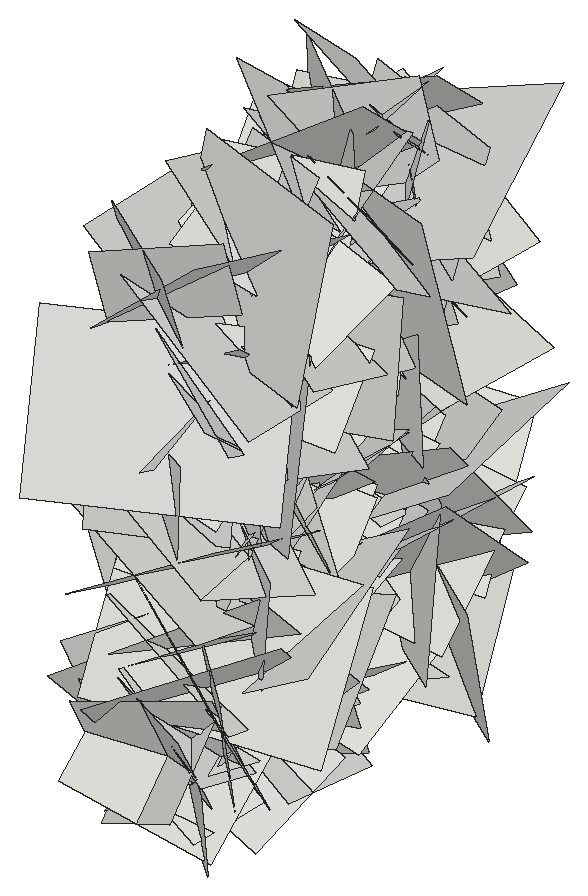
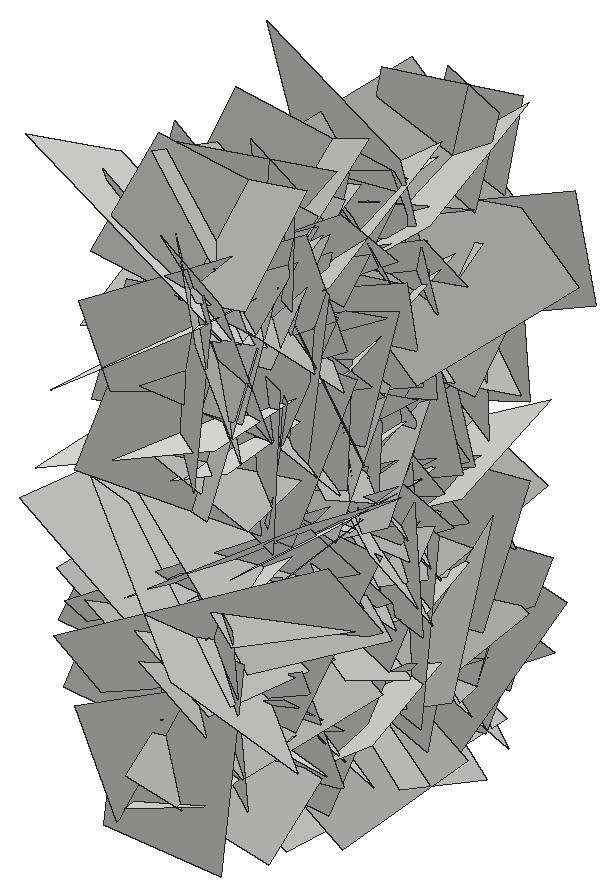
# SketchUp Ruby script. Lengths in inches.
U = 1.inch
M = Sketchup.active_model
def pt(a) = Geom::Point3d.new(a.map { |v| v * U })
def face(e, loops, mat)
  f = e.add_face(loops[0].map { |a| pt(a) })
  loops[1..].each { |l| e.add_face(l.map { |a| pt(a) }).erase! }
  f.material = f.back_material = mat if mat
  f
end
# faces: each face lists its corners as indices into pts; further lists are holes
def faces(e, pts, list, mat = nil) = list.each { |f| face(e, (f[0].is_a?(Array) ? f : [f]).map { |l| l.map { |i| pts[i] } }, mat) }
# xy, xz, yz: faces in a plane at the given z, y or x. An outline is a flat list of corners, or four numbers for a rectangle; further outlines are holes
def ring(l) = l.size == 4 ? [[l[0], l[1]], [l[2], l[1]], [l[2], l[3]], [l[0], l[3]]] : l.each_slice(2).to_a
def flat(e, list, mat, &to3) = list.each { |f| face(e, (f[0].is_a?(Array) ? f : [f]).map { |l| ring(l).map { |u, v| to3.(u, v) } }, mat) }
def xy(e, z, list, mat = nil) = flat(e, list, mat) { |x, y| [x, y, z] }
def xz(e, y, list, mat = nil) = flat(e, list, mat) { |x, z| [x, y, z] }
def yz(e, x, list, mat = nil) = flat(e, list, mat) { |y, z| [x, y, z] }
def lines(e, pts, list) = list.each { |a, b| e.add_line(pt(pts[a]), pt(pts[b])) }
# prism: a flat outline (further loops are holes) pulled along v
def prism(e, loops, v, mat = nil)
  f = face(e, loops, mat); d = Geom::Vector3d.new(v.map { |x| x * U })
  f.pushpull(f.normal.samedirection?(d) ? d.length : -d.length)
end
def box(e, o, s, mat = nil) = prism(e, [[o, [o[0] + s[0], o[1], o[2]], [o[0] + s[0], o[1] + s[1], o[2]], [o[0], o[1] + s[1], o[2]]]], [0, 0, s[2]], mat)
def at(x, y, z, deg = 0) = Geom::Transformation.translation(pt([x, y, z])) * Geom::Transformation.rotation(ORIGIN, Z_AXIS, deg.degrees)
def axes(o, x, y, z) = Geom::Transformation.new([*x, 0, *y, 0, *z, 0, *pt(o).to_a, 1])
def part(name) = M.definitions.add(name)
# library, detail: a bought-in or finely detailed component or shape, given as its bounding box
def library(name, o, s) = part(name).tap { |d| box(d.entities, o, s) }
def detail(e, o, s) = box(e.add_group.entities, o, s)
def put(e, d, t, mat = nil) = e.add_instance(d, t).tap { |i| i.material = mat if mat }
def group(e, t, mat = nil) = e.add_group.tap { |g| g.transformation = t; g.material = mat if mat }.entities
root = M.entities
c1 = part("Component\#6")
p = [[0.01,0,0],[0,3.24,4.54],[4.32,3.24,4.54],[4.33,0,0]]
faces(c1.entities,p,[[0,1,2,3]])
put(root,c1,axes([424.49,182.77,28.15],[0.11013,-1.0722,-0.31704],[0.03816,-0.31503,1.07721],[-1.18456,-0.10983,0.00522]))
put(root,c1,axes([424.49,185.38,28.27],[0.28552,-0.8956,-0.93898],[0.07116,-0.9481,0.92355],[-1.37362,-0.23528,-0.14733]))
put(root,c1,axes([420.52,175.43,34.87],[-0.0411,0.62613,0.35799],[-0.03637,0.3565,-0.62724],[0.76365,0.05068,-0.01061]))
put(root,c1,axes([420.52,173.67,32.24],[-0.05341,-0.65994,-0.37026],[-0.06447,-0.36634,0.66124],[0.79951,-0.07362,0.02859]))
put(root,c1,axes([424.49,174.01,26.46],[0.07872,-0.97306,0.24072],[-0.0738,0.23579,0.97461],[-1.05998,-0.08868,-0.04998]))
put(root,c1,axes([424.49,170.16,39.2],[0.24703,1.2789,-0.21613],[0.13589,-0.24123,-1.28918],[-1.36812,0.20696,-0.16707]))
put(root,c1,axes([420.52,173.15,22.23],[0.01199,-0.5915,0.12784],[0.10227,0.12799,0.58366],[0.63327,-0.00947,-0.09668]))
put(root,c1,axes([420.52,174.375,32.02],[-0.18574,0.64681,-0.5499],[-0.00393,-0.56207,-0.65994],[0.8999,0.13105,-0.11638]))
put(root,c1,axes([420.52,171.42,39.46],[0.01769,0.21401,-0.61924],[0.03571,-0.6189,-0.21298],[0.69357,0.02641,0.02676]))
put(root,c1,axes([420.52,180.11,41],[-0.0874,0.13713,-0.78202],[-0.02965,-0.78624,-0.13492],[0.84107,-0.01347,-0.08602]))
put(root,c1,axes([424.49,182.1,27.04],[0.18817,-1.1788,-0.21223],[0.10509,-0.19936,1.19019],[-1.26526,-0.19187,0.06729]))
put(root,c1,axes([424.49,177.13,31.79],[0.078,-0.30439,1.03044],[0.07955,1.03178,0.29943],[-1.13614,0.05135,0.09171]))
put(root,c1,axes([424.49,172.13,35.78],[-0.07615,0.65901,-0.5201],[-0.04859,-0.52431,-0.658],[-0.88857,-0.02781,0.08055]))
put(root,c1,axes([424.49,172.625,27.43],[0.01975,0.58315,0.74345],[-0.01761,0.74368,-0.58292],[-1.00141,-0.00157,0.02491]))
put(root,c1,axes([424.49,173.5,20.5],[0.29119,-0.77592,0.90535],[-0.00734,0.92801,0.79744],[-1.26387,-0.18415,0.20396]))
put(root,c1,axes([424.49,181.8125,37.17],[0.0246,-0.63961,0.56311],[-0.17949,0.54862,0.63013],[-0.88529,-0.129,-0.11211]))
put(root,c1,axes([420.52,177.7,39.03],[-0.08239,-0.33737,-0.64844],[0.10668,-0.65083,0.32654],[0.76743,0.05425,-0.11501]))
put(root,c1,axes([424.49,176.41,32.2],[-0.11408,-0.0942,-0.79779],[-0.0272,-0.8041,0.09841],[-0.85109,0.03832,0.10379]))
put(root,c1,axes([424.49,171.36,22.89],[-0.02535,0.88672,0.32576],[0.06435,0.32663,-0.88464],[-0.99927,-0.00146,-0.06523]))
put(root,c1,axes([424.49,178.05,19.9375],[0.14578,-1.0409,0.22357],[0.02192,0.228,1.04879],[-1.1283,-0.13006,0.04926]))
put(root,c1,axes([424.49,180.04,24.28],[-0.15161,0.71603,-0.23582],[-0.04269,-0.24694,-0.72538],[-0.79796,-0.12284,0.08362]))
put(root,c1,axes([420.52,173.29,20.87],[0.09428,-0.62013,-0.08152],[0.03551,-0.0775,0.6261],[0.66205,0.09247,-0.02197]))
put(root,c1,axes([420.52,173.36,27.66],[-0.12062,0.63946,0.63128],[-0.06443,0.62939,-0.6485],[0.9503,0.12384,0.03616]))
put(root,c1,axes([424.49,175.14,30.45],[0.22771,0.17317,-1.07869],[-0.0194,-1.09862,-0.18001],[-1.15789,0.05246,-0.20912]))
put(root,c1,axes([424.49,184.3,37.98],[0.01849,-0.42221,-1.00939],[0.24573,-0.98518,0.41609],[-1.13346,-0.22047,0.07374]))
put(root,c1,axes([420.52,172.01,32.68],[0.01531,-0.04852,-0.71126],[0.05574,-0.70939,0.04946],[0.75363,0.05345,0.01079]))
put(root,c1,axes([424.49,172,20.82],[0.19013,-0.4174,1.11707],[0.18593,1.12659,0.39279],[-1.25031,0.10406,0.22828]))
put(root,c1,axes([424.49,178.01,36.42],[-0.04909,-0.68925,0.58112],[0.09024,0.57594,0.68989],[-0.95135,0.0902,0.03545]))
put(root,c1,axes([424.49,174.95,31.63],[-0.12097,-0.07785,-0.70642],[-0.09105,-0.70871,0.09198],[-0.74781,0.09888,0.10307]))
put(root,c1,axes([420.52,171.52,27.71],[-0.03995,0.48298,0.66079],[-0.01207,0.66111,-0.48387],[0.8675,0.03144,0.0237]))
put(root,c1,axes([424.49,174.16,29.86],[-0.19319,0.59277,-0.26834],[-0.07097,-0.29428,-0.60458],[-0.68606,-0.13648,0.1381]))
put(root,c1,axes([424.49,171.18,26.98],[0.09963,0.88743,-0.23237],[-0.05305,-0.22828,-0.89204],[-0.97094,0.10354,0.02489]))
put(root,c1,axes([424.49,169.05,21.98],[-0.04882,0.58162,0.59704],[0.02934,0.59868,-0.58109],[-0.88303,-0.01226,-0.05232]))
put(root,c1,axes([424.49,176.26,32.94],[-0.03084,0.60524,0.59943],[0.03406,0.60013,-0.60439],[-0.90231,0.00196,-0.0433]))
put(root,c1,axes([424.49,174.875,32.24],[-0.12053,0.70886,0.38052],[0.08644,0.39248,-0.70676],[-0.84842,-0.06072,-0.12606]))
put(root,c1,axes([424.49,177.89,30.77],[-0.05678,-0.11721,0.8526],[0.09083,0.84928,0.12214],[-0.90772,0.09231,-0.04111]))
put(root,c1,axes([424.49,177.99,23.55],[-0.04107,0.5427,0.4395],[-0.20397,0.41484,-0.52921],[-0.71159,-0.15024,0.12632]))
put(root,c1,axes([424.49,174.67,32.54],[0.17055,0.3665,0.95024],[0.03456,0.95968,-0.37566],[-1.07902,0.08867,0.13816]))
put(root,c1,axes([424.49,176.52,27.27],[-0.06139,-0.83333,-0.30669],[0.14477,-0.31205,0.82208],[-0.93005,0.00643,0.1482]))
put(root,c1,axes([420.52,180.66,33.34],[-0.08177,-0.45253,0.73357],[0.03972,0.73405,0.45677],[0.91278,-0.07248,0.04584]))
put(root,c1,axes([420.52,181.67,36.78],[-0.05967,0.56874,-0.94691],[-0.29528,-0.9248,-0.5389],[1.13301,-0.21107,-0.19031]))
put(root,c1,axes([420.52,170.91,25.11],[0.00896,0.33986,-0.6335],[0.15678,-0.62081,-0.33108],[0.74574,0.12644,0.07722]))
put(root,c1,axes([424.49,182.09,31.375],[-0.0562,-0.72005,0.10613],[-0.07977,0.11126,0.71729],[-0.76737,0.04117,-0.08234]))
put(root,c1,axes([420.52,175.72,36.8],[-0.15665,0.75943,0.7145],[-0.11122,0.70715,-0.77331],[1.09966,0.17971,0.02357]))
put(root,c1,axes([424.49,175.72,36.8],[0.15665,0.75943,0.7145],[0.11122,0.70715,-0.77331],[-1.09966,0.17971,0.02357]))
put(root,c1,axes([420.52,182.09,31.375],[0.0562,-0.72005,0.10613],[0.07977,0.11126,0.71729],[0.76737,0.04117,-0.08234]))
put(root,c1,axes([424.49,170.91,25.11],[-0.00896,0.33986,-0.6335],[-0.15678,-0.62081,-0.33108],[-0.74574,0.12644,0.07722]))
put(root,c1,axes([424.49,181.67,36.78],[0.05967,0.56874,-0.94691],[0.29528,-0.9248,-0.5389],[-1.13301,-0.21107,-0.19031]))
put(root,c1,axes([424.49,180.66,33.34],[0.08177,-0.45253,0.73357],[-0.03972,0.73405,0.45677],[-0.91278,-0.07248,0.04584]))
put(root,c1,axes([420.52,176.52,27.27],[0.06139,-0.83333,-0.30669],[-0.14477,-0.31205,0.82208],[0.93005,0.00643,0.1482]))
put(root,c1,axes([420.52,174.67,32.54],[-0.17055,0.3665,0.95024],[-0.03456,0.95968,-0.37566],[1.07902,0.08867,0.13816]))
put(root,c1,axes([420.52,177.99,23.55],[0.04107,0.5427,0.4395],[0.20397,0.41484,-0.52921],[0.71159,-0.15024,0.12632]))
put(root,c1,axes([420.52,177.89,30.77],[0.05678,-0.11721,0.8526],[-0.09083,0.84928,0.12214],[0.90772,0.09231,-0.04111]))
put(root,c1,axes([420.52,174.875,32.24],[0.12053,0.70886,0.38052],[-0.08644,0.39248,-0.70676],[0.84842,-0.06072,-0.12606]))
put(root,c1,axes([420.52,176.26,32.94],[0.03084,0.60524,0.59943],[-0.03406,0.60013,-0.60439],[0.90231,0.00196,-0.0433]))
put(root,c1,axes([420.52,169.05,21.98],[0.04882,0.58162,0.59704],[-0.02934,0.59868,-0.58109],[0.88303,-0.01226,-0.05232]))
put(root,c1,axes([420.52,171.18,26.98],[-0.09963,0.88743,-0.23237],[0.05305,-0.22828,-0.89204],[0.97094,0.10354,0.02489]))
put(root,c1,axes([420.52,174.16,29.86],[0.19319,0.59277,-0.26834],[0.07097,-0.29428,-0.60458],[0.68606,-0.13648,0.1381]))
put(root,c1,axes([424.49,171.52,27.71],[0.03995,0.48298,0.66079],[0.01207,0.66111,-0.48387],[-0.8675,0.03144,0.0237]))
put(root,c1,axes([420.52,174.95,31.63],[0.12097,-0.07785,-0.70642],[0.09105,-0.70871,0.09198],[0.74781,0.09888,0.10307]))
put(root,c1,axes([420.52,178.01,36.42],[0.04909,-0.68925,0.58112],[-0.09024,0.57594,0.68989],[0.95135,0.0902,0.03545]))
put(root,c1,axes([420.52,172,20.82],[-0.19013,-0.4174,1.11707],[-0.18593,1.12659,0.39279],[1.25031,0.10406,0.22828]))
put(root,c1,axes([424.49,172.01,32.68],[-0.01531,-0.04852,-0.71126],[-0.05574,-0.70939,0.04946],[-0.75363,0.05345,0.01079]))
put(root,c1,axes([420.52,184.3,37.98],[-0.01849,-0.42221,-1.00939],[-0.24573,-0.98518,0.41609],[1.13346,-0.22047,0.07374]))
put(root,c1,axes([420.52,175.14,30.45],[-0.22771,0.17317,-1.07869],[0.0194,-1.09862,-0.18001],[1.15789,0.05246,-0.20912]))
put(root,c1,axes([424.49,173.36,27.66],[0.12062,0.63946,0.63128],[0.06443,0.62939,-0.6485],[-0.9503,0.12384,0.03616]))
put(root,c1,axes([424.49,173.29,20.87],[-0.09428,-0.62013,-0.08152],[-0.03551,-0.0775,0.6261],[-0.66205,0.09247,-0.02197]))
put(root,c1,axes([420.52,180.04,24.28],[0.15161,0.71603,-0.23582],[0.04269,-0.24694,-0.72538],[0.79796,-0.12284,0.08362]))
put(root,c1,axes([420.52,178.05,19.9375],[-0.14578,-1.0409,0.22357],[-0.02192,0.228,1.04879],[1.1283,-0.13006,0.04926]))
put(root,c1,axes([420.52,171.36,22.89],[0.02535,0.88672,0.32576],[-0.06435,0.32663,-0.88464],[0.99927,-0.00146,-0.06523]))
put(root,c1,axes([420.52,176.41,32.2],[0.11408,-0.0942,-0.79779],[0.0272,-0.8041,0.09841],[0.85109,0.03832,0.10379]))
put(root,c1,axes([424.49,177.7,39.03],[0.08239,-0.33737,-0.64844],[-0.10668,-0.65083,0.32654],[-0.76743,0.05425,-0.11501]))
put(root,c1,axes([420.52,181.8125,37.17],[-0.0246,-0.63961,0.56311],[0.17949,0.54862,0.63013],[0.88529,-0.129,-0.11211]))
put(root,c1,axes([420.52,173.5,20.5],[-0.29119,-0.77592,0.90535],[0.00734,0.92801,0.79744],[1.26387,-0.18415,0.20396]))
put(root,c1,axes([420.52,172.625,27.43],[-0.01975,0.58315,0.74345],[0.01761,0.74368,-0.58292],[1.00141,-0.00157,0.02491]))
put(root,c1,axes([420.52,172.13,35.78],[0.07615,0.65901,-0.5201],[0.04859,-0.52431,-0.658],[0.88857,-0.02781,0.08055]))
put(root,c1,axes([420.52,177.13,31.79],[-0.078,-0.30439,1.03044],[-0.07955,1.03178,0.29943],[1.13614,0.05135,0.09171]))
put(root,c1,axes([420.52,182.1,27.04],[-0.18817,-1.1788,-0.21223],[-0.10509,-0.19936,1.19019],[1.26526,-0.19187,0.06729]))
put(root,c1,axes([424.49,180.11,41],[0.0874,0.13713,-0.78202],[0.02965,-0.78624,-0.13492],[-0.84107,-0.01347,-0.08602]))
put(root,c1,axes([424.49,171.42,39.46],[-0.01769,0.21401,-0.61924],[-0.03571,-0.6189,-0.21298],[-0.69357,0.02641,0.02676]))
put(root,c1,axes([424.49,174.375,32.02],[0.18574,0.64681,-0.5499],[0.00393,-0.56207,-0.65994],[-0.8999,0.13105,-0.11638]))
put(root,c1,axes([420.52,167.34,31.77],[-0.2501,0.51374,1.1242],[-0.05799,1.13903,-0.532],[1.3089,0.14863,0.19123]))
put(root,c1,axes([424.49,173.15,22.23],[-0.01199,-0.5915,0.12784],[-0.10227,0.12799,0.58366],[-0.63327,-0.00947,-0.09668]))
put(root,c1,axes([420.52,170.16,39.2],[-0.24703,1.2789,-0.21613],[-0.13589,-0.24123,-1.28918],[1.36812,0.20696,-0.16707]))
put(root,c1,axes([420.52,174.01,26.46],[-0.07872,-0.97306,0.24072],[0.0738,0.23579,0.97461],[1.05998,-0.08868,-0.04998]))
put(root,c1,axes([424.49,173.67,32.24],[0.05341,-0.65994,-0.37026],[0.06447,-0.36634,0.66124],[-0.79951,-0.07362,0.02859]))
put(root,c1,axes([424.49,175.43,34.87],[0.0411,0.62613,0.35799],[0.03637,0.3565,-0.62724],[-0.76365,0.05068,-0.01061]))
put(root,c1,axes([420.52,185.38,28.27],[-0.28552,-0.8956,-0.93898],[-0.07116,-0.9481,0.92355],[1.37362,-0.23528,-0.14733]))
put(root,c1,axes([420.52,182.77,28.15],[-0.11013,-1.0722,-0.31704],[-0.03816,-0.31503,1.07721],[1.18456,-0.10983,0.00522]))
put(root,c1,axes([420.52,176.05,33.17],[0.01986,0.50916,-0.88553],[-0.06176,-0.8837,-0.50934],[1.08099,-0.05984,-0.01283]))
put(root,c1,axes([424.49,182.27,37.76],[0.22679,0.05489,-0.89691],[0.06736,-0.9206,-0.04118],[-0.95012,-0.05216,-0.217]))
put(root,c1,axes([420.52,174.9,23.69],[-0.06803,0.90477,0.33383],[0.16872,0.33992,-0.89067],[1.00823,0.00417,0.17157]))
put(root,c1,axes([424.49,173.11,21.9],[0.05319,-0.68826,0.19248],[0.04456,0.19546,0.68797],[-0.75624,-0.03689,0.05408]))
put(root,c1,axes([424.49,178.15,33.23],[-0.08938,-0.00525,-0.60269],[0.06829,-0.60515,-0.00374],[-0.63521,-0.06432,0.0844]))
put(root,c1,axes([424.49,176.44,21.6],[0.04345,0.60879,-0.00304],[-0.10651,0.00376,-0.60183],[-0.63647,0.04093,0.10051]))
put(root,c1,axes([420.52,183.67,38.38],[0.04708,0.10578,-1.15378],[-0.2342,-1.13267,-0.11235],[1.2056,-0.22416,0.02323]))
put(root,c1,axes([420.52,173.31,35.98],[-0.01252,1.07454,-0.37217],[-0.12805,-0.37127,-1.06811],[1.19858,-0.02844,-0.11799]))
put(root,c1,axes([420.52,174.78,20.26],[0.10048,-0.39109,0.79293],[0.10042,0.79738,0.38196],[0.93179,-0.04376,-0.12667]))
put(root,c1,axes([424.49,180.68,27.18],[0.06604,-0.60003,0.10008],[-0.10227,0.08959,0.59716],[-0.63666,-0.07663,-0.08554]))
put(root,c1,axes([424.49,170.73,19.61],[0.06378,-0.15247,0.68566],[0.07422,0.68605,0.14641],[-0.74085,0.05561,0.0737]))
put(root,c1,axes([420.52,178.01,21.81],[0.00864,0.40014,0.99077],[-0.02339,0.99065,-0.39991],[1.13239,0.01741,-0.01582]))
put(root,c1,axes([424.49,178.13,40.15],[0.04908,0.64392,0.19174],[0.08573,0.18545,-0.64234],[-0.70699,0.06719,-0.06458]))
put(root,c1,axes([420.52,171.95,33.74],[-0.07102,0.70639,0.8167],[0.11892,0.8184,-0.69866],[1.13841,-0.04142,0.12393]))
put(root,c1,axes([424.49,176.07,37.03],[0.15674,-0.62528,-0.09698],[-0.10666,-0.12156,0.63036],[-0.66219,-0.12843,-0.12449]))
put(root,c1,axes([424.49,180.42,25.12],[0.17902,-0.88337,-0.09354],[0.21931,-0.05348,0.8786],[-0.91571,-0.1855,0.19214]))
put(root,c1,axes([420.52,172.46,21.25],[0.14489,-0.73421,0.72244],[-0.08794,0.71856,0.74596],[1.0883,0.15581,-0.0359]))
put(root,c1,axes([420.52,171.47,32.36],[0.16942,0.96147,-0.31887],[-0.08969,-0.30901,-0.97416],[1.06999,-0.17814,-0.03117]))
put(root,c1,axes([420.52,179.35,38.14],[0.07028,1.07405,0.02302],[-0.04111,0.02544,-1.07534],[1.13802,-0.06541,-0.04027]))
put(root,c1,axes([424.49,181.39,28.46],[0.11732,-0.15238,-0.58962],[-0.01785,-0.59981,0.15186],[-0.64528,-0.01111,-0.1114]))
put(root,c1,axes([424.49,173.74,31.89],[0.15856,-0.67469,0.29232],[0.1064,0.31425,0.67394],[-0.77211,-0.09525,0.1529]))
put(root,c1,axes([420.52,173.84,39.64],[-0.13369,1.27699,-0.41872],[-0.11509,-0.42887,-1.27523],[1.41986,0.08547,-0.14279]))
put(root,c1,axes([424.49,172.58,29],[0.14706,-0.68518,0.03236],[0.10474,0.05263,0.69082],[-0.71951,-0.13238,0.10718]))
put(root,c1,axes([420.52,180.75,35.09],[-0.01445,0.08276,-1.11066],[0.1396,-1.10283,-0.0838],[1.17228,0.13235,-0.00371]))
put(root,c1,axes([420.52,182.25,27.43],[-0.1955,0.46825,-1.21407],[0.10064,-1.21809,-0.48422],[1.37564,0.15566,-0.13711]))
put(root,c1,axes([420.52,175.96,26.52],[0.03553,0.82214,0.9074],[-0.07429,0.90754,-0.81968],[1.2958,0.02948,-0.07187]))
put(root,c1,axes([420.52,172.47,36.95],[0.1233,0.89549,0.4145],[0.21728,0.38634,-0.89217],[1.02316,-0.18996,0.13951]))
put(root,c1,axes([420.52,183.25,38.77],[-0.07927,-0.40868,-1.12281],[0.1988,-1.11508,0.39337],[1.25087,0.15132,-0.13368]))
put(root,c1,axes([420.52,179.04,23.77],[0.11323,-0.75693,-0.7774],[0.09292,-0.77258,0.76428],[1.14637,0.13739,0.01483]))
put(root,c1,axes([420.52,182.77,28.7],[-0.0358,-0.11408,-1.31406],[-0.04325,-1.31377,0.1151],[1.39747,-0.04358,-0.0301]))
put(root,c1,axes([420.52,180.07,24.39],[-0.06666,-0.76105,0.92501],[0.21989,0.90537,0.75899],[1.25053,-0.19976,-0.08415]))
put(root,c1,axes([420.52,177.97,39.67],[-0.02985,0.75948,-0.84861],[0.27983,-0.8214,-0.74388],[1.17429,0.21504,0.15569]))
put(root,c1,axes([420.52,174.06,31.875],[0.08593,-0.00736,1.08266],[0.18405,1.07173,-0.00571],[1.1328,-0.17357,-0.0812]))
put(root,c1,axes([420.52,182.31,23.94],[-0.04872,-1.30982,0.04089],[0.01644,0.04037,1.31055],[1.38898,-0.04642,-0.01408]))
put(root,c1,axes([420.52,178.49,34.59],[0.00763,1.14917,-0.03145],[0.21412,-0.03223,-1.13128],[1.19962,-0.00155,0.20212]))
put(root,c1,axes([420.52,178.09,32.9],[0.18757,-0.47698,-1.21124],[-0.23196,-1.21588,0.44684],[1.36024,-0.14157,0.24323]))
put(root,c1,axes([420.52,178.68,21.25],[0.14964,-1.02559,0.91665],[-0.24358,0.89093,1.03221],[1.43757,0.25771,0.07948]))
put(root,c1,axes([420.52,169.91,24.28],[-0.0494,0.58776,1.07494],[0.25393,1.05932,-0.56884],[1.27358,-0.18841,0.15511]))
put(root,c1,axes([420.52,175.66,39.88],[-0.03914,-0.32872,-1.22009],[0.25418,-1.20026,0.31612],[1.31508,0.2222,-0.09741]))
put(root,c1,axes([420.52,177.96,25.04],[0.10915,-1.1796,-0.55067],[0.03689,-0.5497,1.18402],[1.37942,0.10803,0.01191]))
put(root,c1,axes([420.52,183.77,26.5],[0.0762,-1.33255,-0.21023],[0.04546,-0.20817,1.33413],[1.42926,0.07766,-0.03122]))
put(root,c1,axes([420.52,177.28,39.83],[0.04784,1.11638,-0.64936],[0.22797,-0.64718,-1.09769],[1.34988,0.06974,0.20839]))
put(root,c1,axes([420.52,179.625,37.91],[0.28026,0.12179,-1.29213],[0.26115,-1.29941,-0.07206],[1.35072,0.22596,0.28204]))
put(root,c1,axes([420.52,183.19,37.72],[0.19709,-1.17807,-0.70591],[0.26547,-0.67132,1.18631],[1.43137,0.28672,-0.12282]))
